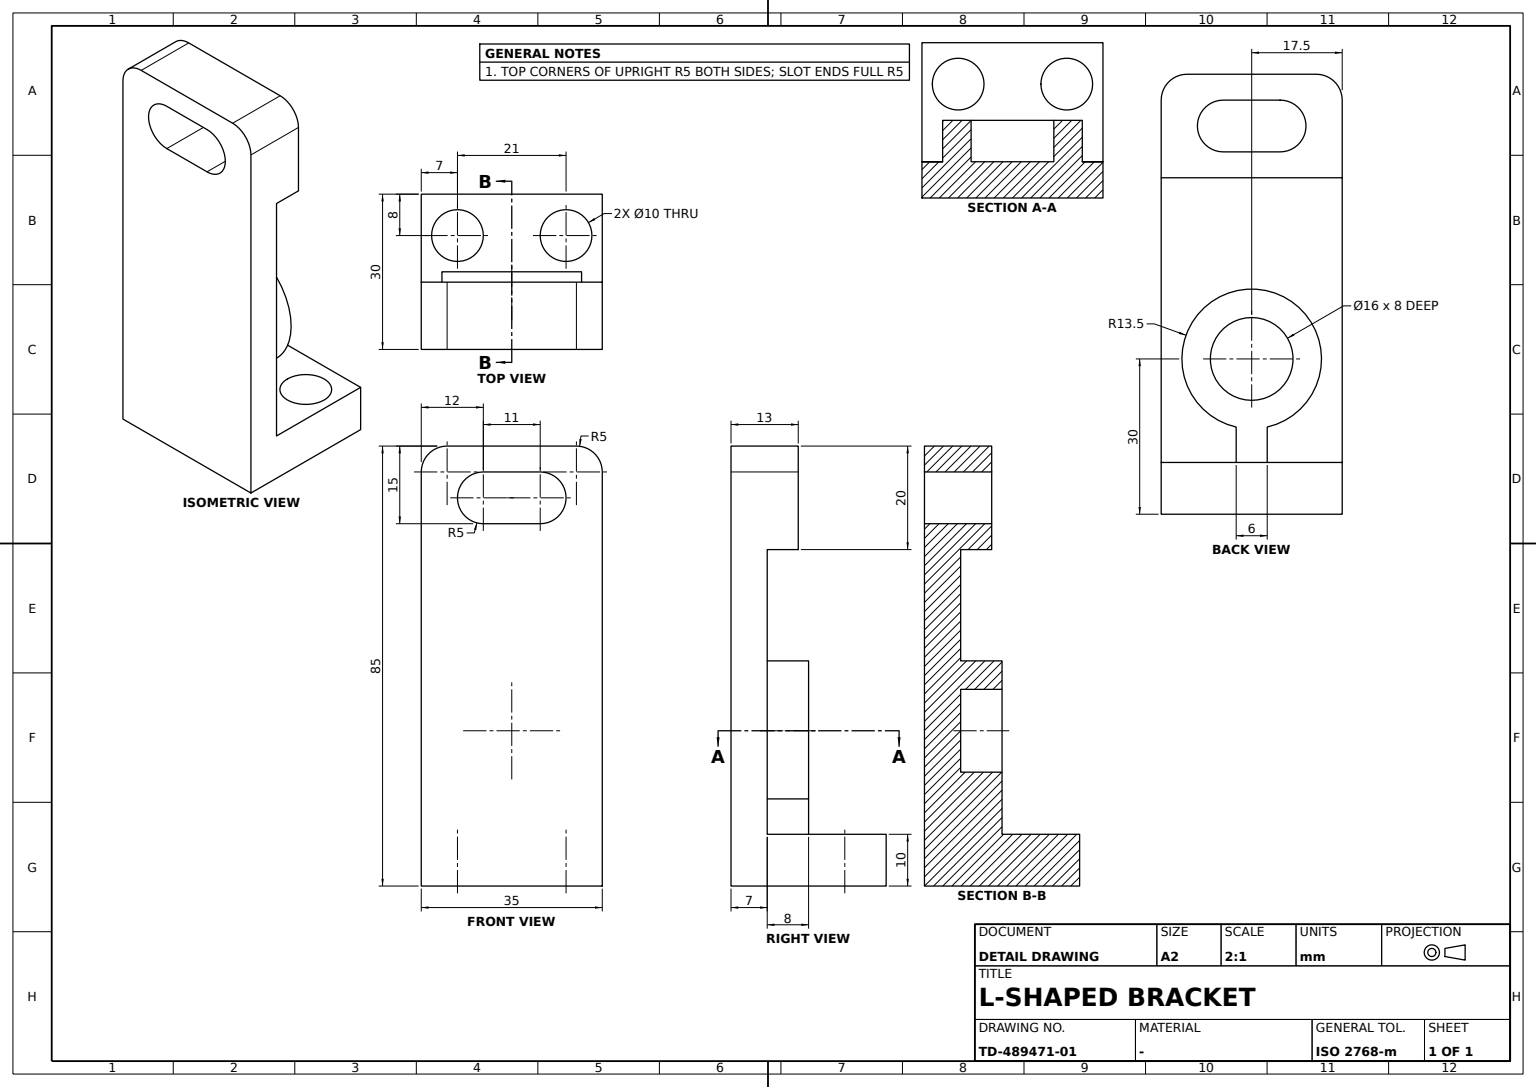
ISO-10303-21;
HEADER;
FILE_DESCRIPTION((''),'2;1');
FILE_NAME('','',(''),(''),'','','');
FILE_SCHEMA(('AUTOMOTIVE_DESIGN'));
ENDSEC;
DATA;
#1=APPLICATION_CONTEXT('');
#2=PRODUCT_CONTEXT('',#1,'mechanical');
#3=PRODUCT('','','',(#2));
#4=PRODUCT_DEFINITION_FORMATION('','',#3);
#5=PRODUCT_DEFINITION_CONTEXT('',#1,'design');
#6=PRODUCT_DEFINITION('','',#4,#5);
#7=PRODUCT_DEFINITION_SHAPE('','',#6);
#8=(LENGTH_UNIT()NAMED_UNIT(*)SI_UNIT(.MILLI.,.METRE.));
#9=(NAMED_UNIT(*)PLANE_ANGLE_UNIT()SI_UNIT($,.RADIAN.));
#10=(NAMED_UNIT(*)SI_UNIT($,.STERADIAN.)SOLID_ANGLE_UNIT());
#11=UNCERTAINTY_MEASURE_WITH_UNIT(LENGTH_MEASURE(0.005),#8,'distance_accuracy_value','');
#12=(GEOMETRIC_REPRESENTATION_CONTEXT(3)GLOBAL_UNCERTAINTY_ASSIGNED_CONTEXT((#11))GLOBAL_UNIT_ASSIGNED_CONTEXT((#8,#9,#10))REPRESENTATION_CONTEXT('',''));
#13=CARTESIAN_POINT('',(3.,7.,16.837553));
#14=VERTEX_POINT('',#13);
#15=CARTESIAN_POINT('',(3.,7.,10.));
#16=VERTEX_POINT('',#15);
#17=DIRECTION('',(0.,0.,-1.));
#18=VECTOR('',#17,1000.);
#19=LINE('',#13,#18);
#20=EDGE_CURVE('',#14,#16,#19,.T.);
#21=ORIENTED_EDGE('',*,*,#20,.T.);
#22=CARTESIAN_POINT('',(3.,15.,10.));
#23=VERTEX_POINT('',#22);
#24=DIRECTION('',(0.,1.,0.));
#25=VECTOR('',#24,1000.);
#26=LINE('',#15,#25);
#27=EDGE_CURVE('',#16,#23,#26,.T.);
#28=ORIENTED_EDGE('',*,*,#27,.T.);
#29=CARTESIAN_POINT('',(3.,15.,16.837553));
#30=VERTEX_POINT('',#29);
#31=CARTESIAN_POINT('',(3.,15.,0.));
#32=LINE('',#31,#18);
#33=EDGE_CURVE('',#30,#23,#32,.T.);
#34=ORIENTED_EDGE('',*,*,#33,.F.);
#35=LINE('',#13,#25);
#36=EDGE_CURVE('',#14,#30,#35,.T.);
#37=ORIENTED_EDGE('',*,*,#36,.F.);
#38=EDGE_LOOP('',(#21,#28,#34,#37));
#39=FACE_BOUND('',#38,.T.);
#40=DIRECTION('',(1.,0.,0.));
#41=AXIS2_PLACEMENT_3D('',#13,#40,#17);
#42=PLANE('',#41);
#43=ADVANCED_FACE('',(#39),#42,.T.);
#44=CARTESIAN_POINT('',(-12.5,0.,85.));
#45=VERTEX_POINT('',#44);
#46=CARTESIAN_POINT('',(-12.5,13.,85.));
#47=VERTEX_POINT('',#46);
#48=CARTESIAN_POINT('',(-12.5,15.,85.));
#49=LINE('',#48,#25);
#50=EDGE_CURVE('',#45,#47,#49,.T.);
#51=ORIENTED_EDGE('',*,*,#50,.F.);
#52=CARTESIAN_POINT('',(12.5,0.,85.));
#53=VERTEX_POINT('',#52);
#54=CARTESIAN_POINT('',(0.,0.,85.));
#55=VECTOR('',#40,1000.);
#56=LINE('',#54,#55);
#57=EDGE_CURVE('',#45,#53,#56,.T.);
#58=ORIENTED_EDGE('',*,*,#57,.T.);
#59=CARTESIAN_POINT('',(12.5,13.,85.));
#60=VERTEX_POINT('',#59);
#61=CARTESIAN_POINT('',(12.5,15.,85.));
#62=LINE('',#61,#25);
#63=EDGE_CURVE('',#53,#60,#62,.T.);
#64=ORIENTED_EDGE('',*,*,#63,.T.);
#65=CARTESIAN_POINT('',(0.,13.,85.));
#66=LINE('',#65,#55);
#67=EDGE_CURVE('',#47,#60,#66,.T.);
#68=ORIENTED_EDGE('',*,*,#67,.F.);
#69=EDGE_LOOP('',(#51,#58,#64,#68));
#70=FACE_BOUND('',#69,.T.);
#71=AXIS2_PLACEMENT_3D('',#54,#17,#24);
#72=PLANE('',#71);
#73=ADVANCED_FACE('',(#70),#72,.F.);
#74=CARTESIAN_POINT('',(-17.5,7.,65.));
#75=VERTEX_POINT('',#74);
#76=CARTESIAN_POINT('',(17.5,7.,65.));
#77=VERTEX_POINT('',#76);
#78=CARTESIAN_POINT('',(0.,7.,65.));
#79=LINE('',#78,#55);
#80=EDGE_CURVE('',#75,#77,#79,.T.);
#81=ORIENTED_EDGE('',*,*,#80,.T.);
#82=CARTESIAN_POINT('',(17.5,7.,10.));
#83=VERTEX_POINT('',#82);
#84=CARTESIAN_POINT('',(17.5,7.,0.));
#85=LINE('',#84,#18);
#86=EDGE_CURVE('',#77,#83,#85,.T.);
#87=ORIENTED_EDGE('',*,*,#86,.T.);
#88=CARTESIAN_POINT('',(0.,7.,10.));
#89=LINE('',#88,#55);
#90=EDGE_CURVE('',#16,#83,#89,.T.);
#91=ORIENTED_EDGE('',*,*,#90,.F.);
#92=ORIENTED_EDGE('',*,*,#20,.F.);
#93=CARTESIAN_POINT('',(-3.,7.,16.837553));
#94=VERTEX_POINT('',#93);
#95=CARTESIAN_POINT('',(0.,7.,30.));
#96=DIRECTION('',(0.,-1.,0.));
#97=AXIS2_PLACEMENT_3D('',#95,#96,#17);
#98=CIRCLE('',#97,13.5);
#99=EDGE_CURVE('',#94,#14,#98,.F.);
#100=ORIENTED_EDGE('',*,*,#99,.F.);
#101=CARTESIAN_POINT('',(-3.,7.,10.));
#102=VERTEX_POINT('',#101);
#103=DIRECTION('',(0.,0.,1.));
#104=VECTOR('',#103,1000.);
#105=LINE('',#101,#104);
#106=EDGE_CURVE('',#102,#94,#105,.T.);
#107=ORIENTED_EDGE('',*,*,#106,.F.);
#108=CARTESIAN_POINT('',(-17.5,7.,10.));
#109=VERTEX_POINT('',#108);
#110=EDGE_CURVE('',#109,#102,#89,.T.);
#111=ORIENTED_EDGE('',*,*,#110,.F.);
#112=CARTESIAN_POINT('',(-17.5,7.,0.));
#113=LINE('',#112,#18);
#114=EDGE_CURVE('',#75,#109,#113,.T.);
#115=ORIENTED_EDGE('',*,*,#114,.F.);
#116=EDGE_LOOP('',(#81,#87,#91,#92,#100,#107,#111,#115));
#117=FACE_BOUND('',#116,.T.);
#118=AXIS2_PLACEMENT_3D('',#78,#96,#17);
#119=PLANE('',#118);
#120=ADVANCED_FACE('',(#117),#119,.F.);
#121=CARTESIAN_POINT('',(-17.5,13.,65.));
#122=VERTEX_POINT('',#121);
#123=CARTESIAN_POINT('',(17.5,13.,65.));
#124=VERTEX_POINT('',#123);
#125=CARTESIAN_POINT('',(0.,13.,65.));
#126=LINE('',#125,#55);
#127=EDGE_CURVE('',#122,#124,#126,.T.);
#128=ORIENTED_EDGE('',*,*,#127,.T.);
#129=CARTESIAN_POINT('',(17.5,0.,65.));
#130=VECTOR('',#96,1000.);
#131=LINE('',#129,#130);
#132=EDGE_CURVE('',#124,#77,#131,.T.);
#133=ORIENTED_EDGE('',*,*,#132,.T.);
#134=ORIENTED_EDGE('',*,*,#80,.F.);
#135=CARTESIAN_POINT('',(-17.5,0.,65.));
#136=LINE('',#135,#130);
#137=EDGE_CURVE('',#122,#75,#136,.T.);
#138=ORIENTED_EDGE('',*,*,#137,.F.);
#139=EDGE_LOOP('',(#128,#133,#134,#138));
#140=FACE_BOUND('',#139,.T.);
#141=AXIS2_PLACEMENT_3D('',#125,#103,#96);
#142=PLANE('',#141);
#143=ADVANCED_FACE('',(#140),#142,.F.);
#144=CARTESIAN_POINT('',(17.5,0.,80.));
#145=VERTEX_POINT('',#144);
#146=CARTESIAN_POINT('',(17.5,13.,80.));
#147=VERTEX_POINT('',#146);
#148=CARTESIAN_POINT('',(17.5,15.,80.));
#149=LINE('',#148,#25);
#150=EDGE_CURVE('',#145,#147,#149,.T.);
#151=ORIENTED_EDGE('',*,*,#150,.T.);
#152=CARTESIAN_POINT('',(12.5,13.,80.));
#153=AXIS2_PLACEMENT_3D('',#152,#96,#17);
#154=CIRCLE('',#153,5.);
#155=EDGE_CURVE('',#147,#60,#154,.T.);
#156=ORIENTED_EDGE('',*,*,#155,.T.);
#157=ORIENTED_EDGE('',*,*,#63,.F.);
#158=CARTESIAN_POINT('',(12.5,0.,80.));
#159=AXIS2_PLACEMENT_3D('',#158,#24,#103);
#160=CIRCLE('',#159,5.);
#161=EDGE_CURVE('',#53,#145,#160,.T.);
#162=ORIENTED_EDGE('',*,*,#161,.T.);
#163=EDGE_LOOP('',(#151,#156,#157,#162));
#164=FACE_BOUND('',#163,.T.);
#165=CARTESIAN_POINT('',(12.5,15.,80.));
#166=AXIS2_PLACEMENT_3D('',#165,#24,#103);
#167=CYLINDRICAL_SURFACE('',#166,5.);
#168=ADVANCED_FACE('',(#164),#167,.T.);
#169=CARTESIAN_POINT('',(17.5,30.,10.));
#170=VERTEX_POINT('',#169);
#171=CARTESIAN_POINT('',(17.5,30.,0.));
#172=VERTEX_POINT('',#171);
#173=LINE('',#171,#18);
#174=EDGE_CURVE('',#170,#172,#173,.T.);
#175=ORIENTED_EDGE('',*,*,#174,.T.);
#176=CARTESIAN_POINT('',(-17.5,30.,0.));
#177=VERTEX_POINT('',#176);
#178=CARTESIAN_POINT('',(0.,30.,0.));
#179=LINE('',#178,#55);
#180=EDGE_CURVE('',#177,#172,#179,.T.);
#181=ORIENTED_EDGE('',*,*,#180,.F.);
#182=CARTESIAN_POINT('',(-17.5,30.,10.));
#183=VERTEX_POINT('',#182);
#184=LINE('',#176,#18);
#185=EDGE_CURVE('',#183,#177,#184,.T.);
#186=ORIENTED_EDGE('',*,*,#185,.F.);
#187=CARTESIAN_POINT('',(0.,30.,10.));
#188=LINE('',#187,#55);
#189=EDGE_CURVE('',#183,#170,#188,.T.);
#190=ORIENTED_EDGE('',*,*,#189,.T.);
#191=EDGE_LOOP('',(#175,#181,#186,#190));
#192=FACE_BOUND('',#191,.T.);
#193=AXIS2_PLACEMENT_3D('',#187,#96,#17);
#194=PLANE('',#193);
#195=ADVANCED_FACE('',(#192),#194,.F.);
#196=CARTESIAN_POINT('',(0.,15.,38.));
#197=VERTEX_POINT('',#196);
#198=CARTESIAN_POINT('',(0.,15.,30.));
#199=AXIS2_PLACEMENT_3D('',#198,#24,#103);
#200=CIRCLE('',#199,8.);
#201=EDGE_CURVE('',#197,#197,#200,.T.);
#202=ORIENTED_EDGE('',*,*,#201,.T.);
#203=EDGE_LOOP('',(#202));
#204=FACE_BOUND('',#203,.T.);
#205=CARTESIAN_POINT('',(0.,7.,22.));
#206=VERTEX_POINT('',#205);
#207=CIRCLE('',#97,8.);
#208=EDGE_CURVE('',#206,#206,#207,.F.);
#209=ORIENTED_EDGE('',*,*,#208,.F.);
#210=EDGE_LOOP('',(#209));
#211=FACE_BOUND('',#210,.T.);
#212=CARTESIAN_POINT('',(0.,11.,30.));
#213=DIRECTION('',(-1.,0.,0.));
#214=AXIS2_PLACEMENT_3D('',#212,#24,#213);
#215=CYLINDRICAL_SURFACE('',#214,8.);
#216=ADVANCED_FACE('',(#204,#211),#215,.F.);
#217=CARTESIAN_POINT('',(5.5,13.,80.));
#218=VERTEX_POINT('',#217);
#219=CARTESIAN_POINT('',(-5.5,13.,80.));
#220=VERTEX_POINT('',#219);
#221=CARTESIAN_POINT('',(0.,13.,80.));
#222=VECTOR('',#213,1000.);
#223=LINE('',#221,#222);
#224=EDGE_CURVE('',#218,#220,#223,.T.);
#225=ORIENTED_EDGE('',*,*,#224,.T.);
#226=CARTESIAN_POINT('',(-5.5,13.,70.));
#227=VERTEX_POINT('',#226);
#228=CARTESIAN_POINT('',(-5.5,13.,75.));
#229=AXIS2_PLACEMENT_3D('',#228,#96,#17);
#230=CIRCLE('',#229,5.);
#231=EDGE_CURVE('',#227,#220,#230,.F.);
#232=ORIENTED_EDGE('',*,*,#231,.F.);
#233=CARTESIAN_POINT('',(5.5,13.,70.));
#234=VERTEX_POINT('',#233);
#235=CARTESIAN_POINT('',(0.,13.,70.));
#236=LINE('',#235,#222);
#237=EDGE_CURVE('',#234,#227,#236,.T.);
#238=ORIENTED_EDGE('',*,*,#237,.F.);
#239=CARTESIAN_POINT('',(5.5,13.,75.));
#240=AXIS2_PLACEMENT_3D('',#239,#96,#17);
#241=CIRCLE('',#240,5.);
#242=EDGE_CURVE('',#218,#234,#241,.F.);
#243=ORIENTED_EDGE('',*,*,#242,.F.);
#244=EDGE_LOOP('',(#225,#232,#238,#243));
#245=FACE_BOUND('',#244,.T.);
#246=CARTESIAN_POINT('',(-17.5,13.,80.));
#247=VERTEX_POINT('',#246);
#248=CARTESIAN_POINT('',(-12.5,13.,80.));
#249=AXIS2_PLACEMENT_3D('',#248,#96,#17);
#250=CIRCLE('',#249,5.);
#251=EDGE_CURVE('',#47,#247,#250,.T.);
#252=ORIENTED_EDGE('',*,*,#251,.F.);
#253=ORIENTED_EDGE('',*,*,#67,.T.);
#254=ORIENTED_EDGE('',*,*,#155,.F.);
#255=CARTESIAN_POINT('',(17.5,13.,0.));
#256=LINE('',#255,#18);
#257=EDGE_CURVE('',#147,#124,#256,.T.);
#258=ORIENTED_EDGE('',*,*,#257,.T.);
#259=ORIENTED_EDGE('',*,*,#127,.F.);
#260=CARTESIAN_POINT('',(-17.5,13.,0.));
#261=LINE('',#260,#18);
#262=EDGE_CURVE('',#247,#122,#261,.T.);
#263=ORIENTED_EDGE('',*,*,#262,.F.);
#264=EDGE_LOOP('',(#252,#253,#254,#258,#259,#263));
#265=FACE_BOUND('',#264,.T.);
#266=AXIS2_PLACEMENT_3D('',#65,#96,#17);
#267=PLANE('',#266);
#268=ADVANCED_FACE('',(#245,#265),#267,.F.);
#269=CARTESIAN_POINT('',(-5.5,0.,70.));
#270=VERTEX_POINT('',#269);
#271=CARTESIAN_POINT('',(-5.5,0.,80.));
#272=VERTEX_POINT('',#271);
#273=CARTESIAN_POINT('',(-5.5,0.,75.));
#274=AXIS2_PLACEMENT_3D('',#273,#24,#103);
#275=CIRCLE('',#274,5.);
#276=EDGE_CURVE('',#270,#272,#275,.T.);
#277=ORIENTED_EDGE('',*,*,#276,.F.);
#278=CARTESIAN_POINT('',(-5.5,5.84,70.));
#279=LINE('',#278,#25);
#280=EDGE_CURVE('',#227,#270,#279,.F.);
#281=ORIENTED_EDGE('',*,*,#280,.F.);
#282=ORIENTED_EDGE('',*,*,#231,.T.);
#283=CARTESIAN_POINT('',(-5.5,5.84,80.));
#284=LINE('',#283,#25);
#285=EDGE_CURVE('',#220,#272,#284,.F.);
#286=ORIENTED_EDGE('',*,*,#285,.T.);
#287=EDGE_LOOP('',(#277,#281,#282,#286));
#288=FACE_BOUND('',#287,.T.);
#289=CARTESIAN_POINT('',(-5.5,5.84,75.));
#290=AXIS2_PLACEMENT_3D('',#289,#24,#213);
#291=CYLINDRICAL_SURFACE('',#290,5.);
#292=ADVANCED_FACE('',(#288),#291,.F.);
#293=CARTESIAN_POINT('',(17.5,0.,0.));
#294=VERTEX_POINT('',#293);
#295=LINE('',#293,#104);
#296=EDGE_CURVE('',#294,#145,#295,.T.);
#297=ORIENTED_EDGE('',*,*,#296,.T.);
#298=ORIENTED_EDGE('',*,*,#161,.F.);
#299=ORIENTED_EDGE('',*,*,#57,.F.);
#300=CARTESIAN_POINT('',(-17.5,0.,80.));
#301=VERTEX_POINT('',#300);
#302=CARTESIAN_POINT('',(-12.5,0.,80.));
#303=AXIS2_PLACEMENT_3D('',#302,#24,#103);
#304=CIRCLE('',#303,5.);
#305=EDGE_CURVE('',#301,#45,#304,.T.);
#306=ORIENTED_EDGE('',*,*,#305,.F.);
#307=CARTESIAN_POINT('',(-17.5,0.,0.));
#308=VERTEX_POINT('',#307);
#309=LINE('',#307,#104);
#310=EDGE_CURVE('',#308,#301,#309,.T.);
#311=ORIENTED_EDGE('',*,*,#310,.F.);
#312=CARTESIAN_POINT('',(0.,0.,0.));
#313=LINE('',#312,#55);
#314=EDGE_CURVE('',#308,#294,#313,.T.);
#315=ORIENTED_EDGE('',*,*,#314,.T.);
#316=EDGE_LOOP('',(#297,#298,#299,#306,#311,#315));
#317=FACE_BOUND('',#316,.T.);
#318=CARTESIAN_POINT('',(5.5,0.,70.));
#319=VERTEX_POINT('',#318);
#320=LINE('',#318,#222);
#321=EDGE_CURVE('',#319,#270,#320,.T.);
#322=ORIENTED_EDGE('',*,*,#321,.T.);
#323=ORIENTED_EDGE('',*,*,#276,.T.);
#324=CARTESIAN_POINT('',(5.5,0.,80.));
#325=VERTEX_POINT('',#324);
#326=LINE('',#324,#222);
#327=EDGE_CURVE('',#325,#272,#326,.T.);
#328=ORIENTED_EDGE('',*,*,#327,.F.);
#329=CARTESIAN_POINT('',(5.5,0.,75.));
#330=AXIS2_PLACEMENT_3D('',#329,#24,#103);
#331=CIRCLE('',#330,5.);
#332=EDGE_CURVE('',#325,#319,#331,.T.);
#333=ORIENTED_EDGE('',*,*,#332,.T.);
#334=EDGE_LOOP('',(#322,#323,#328,#333));
#335=FACE_BOUND('',#334,.T.);
#336=AXIS2_PLACEMENT_3D('',#312,#24,#103);
#337=PLANE('',#336);
#338=ADVANCED_FACE('',(#317,#335),#337,.F.);
#339=ORIENTED_EDGE('',*,*,#285,.F.);
#340=ORIENTED_EDGE('',*,*,#224,.F.);
#341=CARTESIAN_POINT('',(5.5,5.84,80.));
#342=LINE('',#341,#25);
#343=EDGE_CURVE('',#218,#325,#342,.F.);
#344=ORIENTED_EDGE('',*,*,#343,.T.);
#345=ORIENTED_EDGE('',*,*,#327,.T.);
#346=EDGE_LOOP('',(#339,#340,#344,#345));
#347=FACE_BOUND('',#346,.T.);
#348=AXIS2_PLACEMENT_3D('',#217,#103,#213);
#349=PLANE('',#348);
#350=ADVANCED_FACE('',(#347),#349,.F.);
#351=CARTESIAN_POINT('',(17.5,0.,10.));
#352=LINE('',#351,#25);
#353=EDGE_CURVE('',#83,#170,#352,.T.);
#354=ORIENTED_EDGE('',*,*,#353,.F.);
#355=ORIENTED_EDGE('',*,*,#86,.F.);
#356=ORIENTED_EDGE('',*,*,#132,.F.);
#357=ORIENTED_EDGE('',*,*,#257,.F.);
#358=ORIENTED_EDGE('',*,*,#150,.F.);
#359=ORIENTED_EDGE('',*,*,#296,.F.);
#360=LINE('',#293,#130);
#361=EDGE_CURVE('',#172,#294,#360,.T.);
#362=ORIENTED_EDGE('',*,*,#361,.F.);
#363=ORIENTED_EDGE('',*,*,#174,.F.);
#364=EDGE_LOOP('',(#354,#355,#356,#357,#358,#359,#362,#363));
#365=FACE_BOUND('',#364,.T.);
#366=AXIS2_PLACEMENT_3D('',#293,#40,#24);
#367=PLANE('',#366);
#368=ADVANCED_FACE('',(#365),#367,.T.);
#369=CARTESIAN_POINT('',(15.5,22.,0.));
#370=VERTEX_POINT('',#369);
#371=CARTESIAN_POINT('',(10.5,22.,0.));
#372=AXIS2_PLACEMENT_3D('',#371,#103,#40);
#373=CIRCLE('',#372,5.);
#374=EDGE_CURVE('',#370,#370,#373,.T.);
#375=ORIENTED_EDGE('',*,*,#374,.F.);
#376=EDGE_LOOP('',(#375));
#377=FACE_BOUND('',#376,.T.);
#378=CARTESIAN_POINT('',(5.5,22.,10.));
#379=VERTEX_POINT('',#378);
#380=CARTESIAN_POINT('',(10.5,22.,10.));
#381=AXIS2_PLACEMENT_3D('',#380,#17,#213);
#382=CIRCLE('',#381,5.);
#383=EDGE_CURVE('',#379,#379,#382,.F.);
#384=ORIENTED_EDGE('',*,*,#383,.T.);
#385=EDGE_LOOP('',(#384));
#386=FACE_BOUND('',#385,.T.);
#387=CARTESIAN_POINT('',(10.5,22.,1.25));
#388=AXIS2_PLACEMENT_3D('',#387,#103,#24);
#389=CYLINDRICAL_SURFACE('',#388,5.);
#390=ADVANCED_FACE('',(#377,#386),#389,.F.);
#391=CARTESIAN_POINT('',(-17.5,15.,80.));
#392=LINE('',#391,#25);
#393=EDGE_CURVE('',#301,#247,#392,.T.);
#394=ORIENTED_EDGE('',*,*,#393,.T.);
#395=ORIENTED_EDGE('',*,*,#262,.T.);
#396=ORIENTED_EDGE('',*,*,#137,.T.);
#397=ORIENTED_EDGE('',*,*,#114,.T.);
#398=CARTESIAN_POINT('',(-17.5,0.,10.));
#399=LINE('',#398,#25);
#400=EDGE_CURVE('',#109,#183,#399,.T.);
#401=ORIENTED_EDGE('',*,*,#400,.T.);
#402=ORIENTED_EDGE('',*,*,#185,.T.);
#403=LINE('',#307,#130);
#404=EDGE_CURVE('',#177,#308,#403,.T.);
#405=ORIENTED_EDGE('',*,*,#404,.T.);
#406=ORIENTED_EDGE('',*,*,#310,.T.);
#407=EDGE_LOOP('',(#394,#395,#396,#397,#401,#402,#405,#406));
#408=FACE_BOUND('',#407,.T.);
#409=AXIS2_PLACEMENT_3D('',#307,#40,#24);
#410=PLANE('',#409);
#411=ADVANCED_FACE('',(#408),#410,.F.);
#412=ORIENTED_EDGE('',*,*,#99,.T.);
#413=ORIENTED_EDGE('',*,*,#36,.T.);
#414=CARTESIAN_POINT('',(-3.,15.,16.837553));
#415=VERTEX_POINT('',#414);
#416=CIRCLE('',#199,13.5);
#417=EDGE_CURVE('',#415,#30,#416,.T.);
#418=ORIENTED_EDGE('',*,*,#417,.F.);
#419=LINE('',#93,#25);
#420=EDGE_CURVE('',#94,#415,#419,.T.);
#421=ORIENTED_EDGE('',*,*,#420,.F.);
#422=EDGE_LOOP('',(#412,#413,#418,#421));
#423=FACE_BOUND('',#422,.T.);
#424=CYLINDRICAL_SURFACE('',#214,13.5);
#425=ADVANCED_FACE('',(#423),#424,.T.);
#426=CARTESIAN_POINT('',(-3.,15.,10.));
#427=VERTEX_POINT('',#426);
#428=CARTESIAN_POINT('',(0.,15.,10.));
#429=LINE('',#428,#222);
#430=EDGE_CURVE('',#23,#427,#429,.T.);
#431=ORIENTED_EDGE('',*,*,#430,.T.);
#432=CARTESIAN_POINT('',(-3.,15.,0.));
#433=LINE('',#432,#104);
#434=EDGE_CURVE('',#427,#415,#433,.T.);
#435=ORIENTED_EDGE('',*,*,#434,.T.);
#436=ORIENTED_EDGE('',*,*,#417,.T.);
#437=ORIENTED_EDGE('',*,*,#33,.T.);
#438=EDGE_LOOP('',(#431,#435,#436,#437));
#439=FACE_BOUND('',#438,.T.);
#440=ORIENTED_EDGE('',*,*,#201,.F.);
#441=EDGE_LOOP('',(#440));
#442=FACE_BOUND('',#441,.T.);
#443=CARTESIAN_POINT('',(0.,15.,0.));
#444=AXIS2_PLACEMENT_3D('',#443,#24,#213);
#445=PLANE('',#444);
#446=ADVANCED_FACE('',(#439,#442),#445,.T.);
#447=ORIENTED_EDGE('',*,*,#50,.T.);
#448=ORIENTED_EDGE('',*,*,#251,.T.);
#449=ORIENTED_EDGE('',*,*,#393,.F.);
#450=ORIENTED_EDGE('',*,*,#305,.T.);
#451=EDGE_LOOP('',(#447,#448,#449,#450));
#452=FACE_BOUND('',#451,.T.);
#453=CARTESIAN_POINT('',(-12.5,15.,80.));
#454=AXIS2_PLACEMENT_3D('',#453,#24,#213);
#455=CYLINDRICAL_SURFACE('',#454,5.);
#456=ADVANCED_FACE('',(#452),#455,.T.);
#457=ORIENTED_EDGE('',*,*,#208,.T.);
#458=EDGE_LOOP('',(#457));
#459=FACE_BOUND('',#458,.T.);
#460=ADVANCED_FACE('',(#459),#119,.F.);
#461=CARTESIAN_POINT('',(-15.5,22.,10.));
#462=VERTEX_POINT('',#461);
#463=CARTESIAN_POINT('',(-10.5,22.,10.));
#464=AXIS2_PLACEMENT_3D('',#463,#17,#213);
#465=CIRCLE('',#464,5.);
#466=EDGE_CURVE('',#462,#462,#465,.F.);
#467=ORIENTED_EDGE('',*,*,#466,.T.);
#468=EDGE_LOOP('',(#467));
#469=FACE_BOUND('',#468,.T.);
#470=CARTESIAN_POINT('',(-5.5,22.,0.));
#471=VERTEX_POINT('',#470);
#472=CARTESIAN_POINT('',(-10.5,22.,0.));
#473=AXIS2_PLACEMENT_3D('',#472,#103,#40);
#474=CIRCLE('',#473,5.);
#475=EDGE_CURVE('',#471,#471,#474,.T.);
#476=ORIENTED_EDGE('',*,*,#475,.F.);
#477=EDGE_LOOP('',(#476));
#478=FACE_BOUND('',#477,.T.);
#479=CARTESIAN_POINT('',(-10.5,22.,1.25));
#480=AXIS2_PLACEMENT_3D('',#479,#103,#24);
#481=CYLINDRICAL_SURFACE('',#480,5.);
#482=ADVANCED_FACE('',(#469,#478),#481,.F.);
#483=ORIENTED_EDGE('',*,*,#374,.T.);
#484=EDGE_LOOP('',(#483));
#485=FACE_BOUND('',#484,.T.);
#486=ORIENTED_EDGE('',*,*,#475,.T.);
#487=EDGE_LOOP('',(#486));
#488=FACE_BOUND('',#487,.T.);
#489=ORIENTED_EDGE('',*,*,#361,.T.);
#490=ORIENTED_EDGE('',*,*,#314,.F.);
#491=ORIENTED_EDGE('',*,*,#404,.F.);
#492=ORIENTED_EDGE('',*,*,#180,.T.);
#493=EDGE_LOOP('',(#489,#490,#491,#492));
#494=FACE_BOUND('',#493,.T.);
#495=AXIS2_PLACEMENT_3D('',#178,#103,#96);
#496=PLANE('',#495);
#497=ADVANCED_FACE('',(#485,#488,#494),#496,.F.);
#498=ORIENTED_EDGE('',*,*,#466,.F.);
#499=EDGE_LOOP('',(#498));
#500=FACE_BOUND('',#499,.T.);
#501=ORIENTED_EDGE('',*,*,#430,.F.);
#502=ORIENTED_EDGE('',*,*,#27,.F.);
#503=ORIENTED_EDGE('',*,*,#90,.T.);
#504=ORIENTED_EDGE('',*,*,#353,.T.);
#505=ORIENTED_EDGE('',*,*,#189,.F.);
#506=ORIENTED_EDGE('',*,*,#400,.F.);
#507=ORIENTED_EDGE('',*,*,#110,.T.);
#508=LINE('',#101,#25);
#509=EDGE_CURVE('',#102,#427,#508,.T.);
#510=ORIENTED_EDGE('',*,*,#509,.T.);
#511=EDGE_LOOP('',(#501,#502,#503,#504,#505,#506,#507,#510));
#512=FACE_BOUND('',#511,.T.);
#513=ORIENTED_EDGE('',*,*,#383,.F.);
#514=EDGE_LOOP('',(#513));
#515=FACE_BOUND('',#514,.T.);
#516=AXIS2_PLACEMENT_3D('',#88,#17,#24);
#517=PLANE('',#516);
#518=ADVANCED_FACE('',(#500,#512,#515),#517,.F.);
#519=ORIENTED_EDGE('',*,*,#434,.F.);
#520=ORIENTED_EDGE('',*,*,#509,.F.);
#521=ORIENTED_EDGE('',*,*,#106,.T.);
#522=ORIENTED_EDGE('',*,*,#420,.T.);
#523=EDGE_LOOP('',(#519,#520,#521,#522));
#524=FACE_BOUND('',#523,.T.);
#525=AXIS2_PLACEMENT_3D('',#101,#213,#103);
#526=PLANE('',#525);
#527=ADVANCED_FACE('',(#524),#526,.T.);
#528=CARTESIAN_POINT('',(5.5,5.84,70.));
#529=LINE('',#528,#25);
#530=EDGE_CURVE('',#234,#319,#529,.F.);
#531=ORIENTED_EDGE('',*,*,#530,.F.);
#532=ORIENTED_EDGE('',*,*,#237,.T.);
#533=ORIENTED_EDGE('',*,*,#280,.T.);
#534=ORIENTED_EDGE('',*,*,#321,.F.);
#535=EDGE_LOOP('',(#531,#532,#533,#534));
#536=FACE_BOUND('',#535,.T.);
#537=AXIS2_PLACEMENT_3D('',#233,#103,#213);
#538=PLANE('',#537);
#539=ADVANCED_FACE('',(#536),#538,.T.);
#540=ORIENTED_EDGE('',*,*,#530,.T.);
#541=ORIENTED_EDGE('',*,*,#332,.F.);
#542=ORIENTED_EDGE('',*,*,#343,.F.);
#543=ORIENTED_EDGE('',*,*,#242,.T.);
#544=EDGE_LOOP('',(#540,#541,#542,#543));
#545=FACE_BOUND('',#544,.T.);
#546=CARTESIAN_POINT('',(5.5,5.84,75.));
#547=AXIS2_PLACEMENT_3D('',#546,#24,#213);
#548=CYLINDRICAL_SURFACE('',#547,5.);
#549=ADVANCED_FACE('',(#545),#548,.F.);
#550=CLOSED_SHELL('',(#43,#73,#120,#143,#168,#195,#216,#268,#292,#338,#350,#368,#390,#411,#425,#446,#456,#460,#482,#497,#518,#527,#539,#549));
#551=MANIFOLD_SOLID_BREP('',#550);
#552=ADVANCED_BREP_SHAPE_REPRESENTATION('',(#551),#12);
#553=SHAPE_DEFINITION_REPRESENTATION(#7,#552);
ENDSEC;
END-ISO-10303-21;
